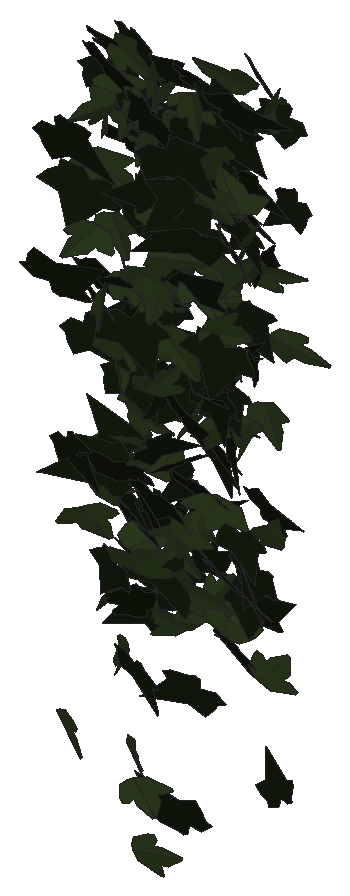
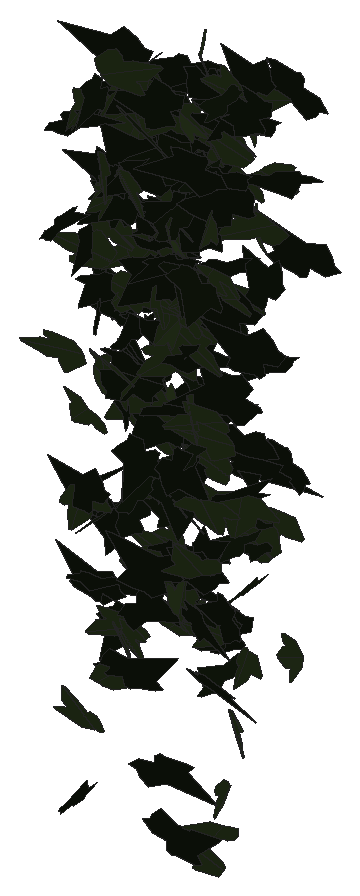
# SketchUp Ruby script. Lengths in millimetres.
U = 1.mm
M = Sketchup.active_model
def pt(a) = Geom::Point3d.new(a.map { |v| v * U })
def face(e, loops, mat)
  f = e.add_face(loops[0].map { |a| pt(a) })
  loops[1..].each { |l| e.add_face(l.map { |a| pt(a) }).erase! }
  f.material = f.back_material = mat if mat
  f
end
# faces: each face lists its corners as indices into pts; further lists are holes
def faces(e, pts, list, mat = nil) = list.each { |f| face(e, (f[0].is_a?(Array) ? f : [f]).map { |l| l.map { |i| pts[i] } }, mat) }
# xy, xz, yz: faces in a plane at the given z, y or x. An outline is a flat list of corners, or four numbers for a rectangle; further outlines are holes
def ring(l) = l.size == 4 ? [[l[0], l[1]], [l[2], l[1]], [l[2], l[3]], [l[0], l[3]]] : l.each_slice(2).to_a
def flat(e, list, mat, &to3) = list.each { |f| face(e, (f[0].is_a?(Array) ? f : [f]).map { |l| ring(l).map { |u, v| to3.(u, v) } }, mat) }
def xy(e, z, list, mat = nil) = flat(e, list, mat) { |x, y| [x, y, z] }
def xz(e, y, list, mat = nil) = flat(e, list, mat) { |x, z| [x, y, z] }
def yz(e, x, list, mat = nil) = flat(e, list, mat) { |y, z| [x, y, z] }
def lines(e, pts, list) = list.each { |a, b| e.add_line(pt(pts[a]), pt(pts[b])) }
# prism: a flat outline (further loops are holes) pulled along v
def prism(e, loops, v, mat = nil)
  f = face(e, loops, mat); d = Geom::Vector3d.new(v.map { |x| x * U })
  f.pushpull(f.normal.samedirection?(d) ? d.length : -d.length)
end
def box(e, o, s, mat = nil) = prism(e, [[o, [o[0] + s[0], o[1], o[2]], [o[0] + s[0], o[1] + s[1], o[2]], [o[0], o[1] + s[1], o[2]]]], [0, 0, s[2]], mat)
def at(x, y, z, deg = 0) = Geom::Transformation.translation(pt([x, y, z])) * Geom::Transformation.rotation(ORIGIN, Z_AXIS, deg.degrees)
def axes(o, x, y, z) = Geom::Transformation.new([*x, 0, *y, 0, *z, 0, *pt(o).to_a, 1])
def part(name) = M.definitions.add(name)
# library, detail: a bought-in or finely detailed component or shape, given as its bounding box
def library(name, o, s) = part(name).tap { |d| box(d.entities, o, s) }
def detail(e, o, s) = box(e.add_group.entities, o, s)
def put(e, d, t, mat = nil) = e.add_instance(d, t).tap { |i| i.material = mat if mat }
def group(e, t, mat = nil) = e.add_group.tap { |g| g.transformation = t; g.material = mat if mat }.entities
root = M.entities
M.materials.add("efeu1").color = [18, 25, 13]
M.materials.add("efeu2").color = [43, 57, 29]
c1 = part("ivyleaf_10")
p = [[0,12.8,-0.8],[-1.5,51.3,-10.9],[-4.9,51,-11.6],[-13.6,26.5,-7.3],[-13.2,15.9,-4.6],[-21.1,19.3,-7.2],
  [-29.5,16.3,-8.3],[-29.2,8.3,-6.2],[-19.7,-9.8,0.5],[-7.6,-13,4],[1,-12.2,5.8],[-0.4,51.1,-11.1],
  [-1.5,51.1,-10.9],[1,-12.4,5.9],[16.9,-12.4,3.5],[35.1,9.1,-5.1],[35,12.9,-6.1],[20.5,16.4,-4.9],
  [15.8,15,-3.8],[15.3,27.6,-7.1],[12.8,31.3,-7.8]]
faces(c1.entities,p,[[0,1,2,3,4,5,6,7,8,9,10],[11,12,0,13,14,15,16,17,18,19,20]],"efeu2")
c2 = part("ivyleaf_9")
p = [[39.1,54.8,31.7],[34.5,51.8,30.2],[-5.3,25.2,17.3],[-17.9,28.3,20.9],[-21.6,21.7,17],[-20.2,4.3,5.3],
  [-22.9,-0.3,2.5],[-17.1,-4,-0.6],[-2,-2.1,-1.2],[-0.7,-15.4,-10.1],[16.6,-22.3,-16.7],[21.1,-15.1,-12.5],
  [32.7,-10.7,-11],[46.1,-1.8,-6.6],[30.8,11.2,3.8]]
faces(c2.entities,p,[[0,1,2,3,4,5,6,7,8,9,10,11,12,13,14]],"efeu1")
put(root,c1,axes([3656.9,861.6,676],[-0.21745,-0.61907,-0.70388],[0.25823,0.6907,-0.6295],[1.76524,-0.1773,0.00538]))
put(root,c2,axes([3619.2,879.4,1196],[0.43031,-0.2889,0.97302],[1.40578,-0.6369,-0.36074],[1.32495,0.76958,0.06673]))
put(root,c2,axes([3622.1,885.5,1606.1],[1.16583,-0.45712,0.56824],[0.91117,-0.30774,-0.76366],[1.04702,0.7768,0.03186]))
put(root,c2,axes([3630,936,783.7],[0.2375,-0.07977,-0.92172],[1.74289,-0.12157,0.1345],[-0.25033,-0.92215,0.062]))
put(root,c1,axes([3628.2,860,1412.2],[1.26885,0.39586,0.80002],[1.29166,0.42377,-0.77526],[-1.10342,0.95128,0.01245]))
put(root,c2,axes([3691.3,953.1,779.3],[-0.34759,0.04433,-0.93711],[-1.77378,0.10065,0.1864],[0.20427,0.94942,0.02399]))
put(root,c1,axes([3663.2,952.2,969.9],[1.67301,0.22774,-0.19223],[-0.3649,-0.02621,-0.9078],[-0.43424,0.89944,0.02222]))
put(root,c1,axes([3666.5,866.2,935.9],[-1.58811,-0.58537,-0.12744],[0.19729,0.07413,-1.01929],[1.12296,-0.84085,-0.00115]))
put(root,c1,axes([3673.5,872.7,571.9],[0.46708,-0.7584,-0.53558],[-0.31943,0.50861,-0.79712],[1.73792,0.29731,-0.00257]))
put(root,c1,axes([3666.9,934.4,1435.8],[0.00493,-0.38442,-0.8398],[0.11088,0.8382,-0.3835],[1.7543,-0.0519,0.0266]))
put(root,c2,axes([3638.2,847.8,875.4],[1.2816,-0.59575,0.122],[0.18383,-0.07494,-0.89907],[1.14267,0.68024,0.00781]))
put(root,c1,axes([3635.4,851.2,863],[-0.96122,-0.02168,0.90204],[1.71102,-0.10013,0.50096],[0.14625,1.02895,0.06776]))
put(root,c2,axes([3671,956.2,1340.8],[0.44979,0.87871,0.40823],[0.22838,0.39042,-0.90984],[-1.82983,0.26472,-0.01321]))
put(root,c2,axes([3687.5,868.9,933.3],[-1.18232,-0.80256,0.2106],[0.27947,0.15259,1.01465],[-1.55421,0.63796,0.02225]))
put(root,c2,axes([3648.9,813.2,1155.2],[0.37024,-0.72384,-0.70986],[-0.01983,0.72135,-0.7384],[1.92942,0.14631,0.12863]))
put(root,c2,axes([3649.4,866.1,1584.9],[-0.1163,-0.61134,-0.73367],[0.43346,0.70463,-0.60611],[1.7651,-0.21332,0.1005]))
put(root,c2,axes([3646.6,773.1,969.1],[-0.38652,-0.0196,-0.94676],[1.8015,0.02388,-0.20354],[0.05227,-0.968,0.01415]))
put(root,c2,axes([3657.1,922.1,1515],[-0.24426,-0.59721,-0.69735],[0.33536,0.67502,-0.61051],[1.71489,-0.21707,0.02006]))
put(root,c2,axes([3645.4,891.3,1130.4],[1.6713,0.14103,0.51566],[0.97157,0.07319,-0.88937],[-0.30206,1.01572,-0.00751]))
put(root,c2,axes([3703.3,907.6,645.4],[-1.69308,0.2827,0.00809],[-0.01696,-0.00134,-0.93343],[-0.53798,-0.88963,0.00397]))
put(root,c2,axes([3687.4,954.7,1351.5],[0.39695,0.8879,0.40846],[0.19909,0.39498,-0.91201],[-1.8494,0.2331,-0.01051]))
put(root,c1,axes([3649.4,936.1,1074.4],[-0.21937,-0.08976,-0.936],[1.77507,-0.13076,-0.10232],[-0.22743,-0.93397,0.10429]))
put(root,c1,axes([3662.9,916.4,735.4],[0.85517,0.18966,-0.7966],[1.12189,0.55578,0.46483],[1.08175,-0.72634,0.14767]))
put(root,c2,axes([3661.9,905.7,1623],[0.65898,-0.84368,0.2148],[0.1378,-0.20245,-0.91192],[1.65117,0.35361,-0.00962]))
put(root,c2,axes([3655.9,722.2,1275.2],[-0.47995,0.04865,1.02424],[1.56186,-0.62281,0.23164],[1.17005,0.85133,0.11093]))
put(root,c2,axes([3686.8,771,1434.7],[-1.28367,-0.88403,-0.01548],[0.0178,0.01233,-1.11195],[1.68265,-0.67454,-0.00004]))
put(root,c2,axes([3659,964.6,1541.7],[0.20429,0.13717,-0.89428],[1.09147,0.6862,0.17409],[1.33178,-0.58343,-0.0055]))
put(root,c2,axes([3664.1,863.8,865.9],[0.7315,-0.89886,0.23349],[0.23371,-0.20129,-0.97703],[1.75196,0.40216,0.03285]))
put(root,c1,axes([3682.6,770.3,862.1],[-1.35554,-0.58375,-0.47634],[0.76287,0.26145,-0.91974],[1.21417,-0.81599,0.04607]))
put(root,c2,axes([3729.3,792,946.7],[-1.83934,-0.13213,0.57145],[-1.07745,-0.0778,-0.97544],[0.29182,-1.12005,0.00034]))
put(root,c1,axes([3665.9,934.9,1102.2],[0.61249,0.27061,0.85149],[1.14987,0.60083,-0.4193],[-1.25271,0.68382,0.03144]))
put(root,c1,axes([3677.7,951.3,856.5],[1.28464,0.44572,-0.49084],[0.78541,0.26579,0.80886],[0.98762,-0.79113,-0.00479]))
put(root,c2,axes([3704.5,973,1036.4],[-0.4994,0.64473,-0.79081],[0.56615,-0.73273,-0.69608],[-1.85752,-0.39666,0.00046]))
put(root,c1,axes([3702.2,792.3,1564.2],[0.02712,-0.18041,1.09376],[-0.03713,-1.09372,-0.18015],[2.10945,-0.01693,-0.01723]))
put(root,c2,axes([3664.1,895.3,1439.8],[1.99242,0.11403,-0.23279],[0.43455,0.05293,1.05272],[0.23357,-1.07114,0.02724]))
put(root,c1,axes([3692.4,844.7,1098],[-0.04657,0.87777,-0.46591],[0.00724,-0.46597,-0.87807],[-1.8913,-0.0234,0.00811]))
put(root,c2,axes([3671.8,824,1610.1],[0.1947,-0.36131,0.95831],[0.7325,-0.87892,-0.37247],[1.80631,0.39537,0.04775]))
put(root,c1,axes([3676,848.3,1570.1],[1.23771,0.43203,0.5737],[0.9251,0.30496,-0.78066],[-1.00619,0.81182,-0.01205]))
put(root,c1,axes([3683.2,814.1,1532.5],[-0.20584,0.08717,0.99849],[1.16609,-0.78903,0.13525],[1.50962,0.62137,0.03167]))
put(root,c2,axes([3685.5,938.1,1499.9],[-0.06883,-0.70313,0.65646],[0.13713,-0.65706,-0.6998],[1.82563,0.02284,0.07732]))
put(root,c1,axes([3695.4,921.7,1306],[0.0097,0.27879,0.91595],[0.05528,0.9155,-0.27881],[-1.82136,0.02927,-0.00358]))
put(root,c1,axes([3706.7,931.7,1114],[0.35004,-0.95221,-0.29135],[-0.01287,0.29508,-0.96866],[1.89514,0.17788,0.04724]))
put(root,c2,axes([3699.2,821.4,751.9],[-0.36075,-0.63647,0.63104],[-0.27021,-0.61553,-0.66348],[1.68425,-0.23508,0.02872]))
put(root,c1,axes([3672.8,865.5,1620.4],[0.52665,-0.04353,0.97521],[1.8006,-0.23776,-0.27907],[0.4577,0.98543,-0.02426]))
put(root,c1,axes([3740.6,906.9,1202.3],[-1.08951,0.04027,0.78396],[-1.49041,-0.0966,-0.56687],[0.10363,-0.96591,0.08937]))
put(root,c2,axes([3676.7,896.9,723.2],[0.67271,-0.64871,0.71095],[0.73097,-0.59938,-0.73786],[1.67952,0.5207,0.03638]))
put(root,c2,axes([3693.9,855.8,1072.6],[0.16033,-0.92547,-0.48982],[-0.09594,0.48724,-0.92928],[1.99053,0.09803,-0.00534]))
put(root,c1,axes([3711.4,847.1,428],[-0.78238,0.78469,0.13375],[-0.12398,0.11687,-0.88585],[-1.50989,-0.4162,0.00343]))
put(root,c2,axes([3732.9,912.1,1182.4],[-0.12547,-0.31972,-0.89004],[-0.34126,-0.8718,0.32644],[-1.76726,0.19104,0.00015]))
put(root,c2,axes([3690.2,945.3,1040.6],[0.81623,-0.84097,0.0972],[0.08586,-0.0861,-0.94402],[1.60891,0.43124,0.00106]))
put(root,c2,axes([3688.9,776.2,1239.5],[0.16706,-0.43073,1.07078],[0.44133,-1.0454,-0.43952],[2.15182,0.24785,0.00701]))
put(root,c1,axes([3677.6,863.5,1518.4],[0.8567,-0.25701,-1.03394],[1.92297,-0.25306,0.50279],[-0.64319,-1.09892,0.12603]))
put(root,c2,axes([3742.3,870.1,1549.8],[-0.28626,-0.38716,-0.88076],[-0.404,-0.85613,0.41259],[-1.78594,0.25572,0.04784]))
put(root,c1,axes([3718,831.1,1541.5],[1.22018,-0.65683,0.09752],[0.12784,-0.07071,-0.91786],[1.2573,0.64463,-0.00131]))
put(root,c2,axes([3730.5,793.1,1187.6],[0.14784,0.5784,0.83399],[0.2192,0.826,-0.58359],[-1.91914,0.1389,-0.00241]))
put(root,c2,axes([3737.7,866.9,819.1],[0.10398,-0.51843,0.78811],[-0.23867,0.77843,0.52076],[-1.77943,-0.13471,-0.02379]))
put(root,c2,axes([3684.4,702.3,1555],[-0.00715,-0.1984,-1.09862],[2.03355,0.31772,-0.06103],[0.6157,-1.05168,0.18881]))
put(root,c2,axes([3706.5,970.2,1374.1],[0.2403,-0.54117,-0.7389],[0.10151,0.74896,-0.53943],[1.74014,0.03104,0.1335]))
put(root,c1,axes([3719.6,867,1484],[1.28921,-0.66424,0.18482],[0.25333,-0.12824,-0.94872],[1.28753,0.69034,0.0016]))
put(root,c1,axes([3694.3,877.1,986.3],[-0.29166,-0.01332,0.92108],[1.73339,-0.1421,0.14948],[0.26269,0.92287,0.03631]))
put(root,c2,axes([3755,950.4,501.9],[0.1189,0.05227,-0.90793],[-1.14396,-0.68058,-0.08054],[-1.29889,0.60419,-0.01218]))
put(root,c1,axes([3718.9,852.3,362.4],[0.99501,0.70498,0.2678],[0.30626,0.21407,-0.87768],[-1.4022,0.54701,-0.00166]))
put(root,c1,axes([3742.6,710.9,1393.5],[0.95573,0.5619,-0.68683],[-0.86734,-0.51386,-0.7536],[-1.44916,0.67813,-0.00193]))
put(root,c2,axes([3743.1,762.5,972.7],[1.20316,0.47432,-0.58118],[-0.94156,-0.30772,-0.78927],[-1.07323,0.80171,0.0409]))
put(root,c2,axes([3707.1,829,685.7],[0.5167,0.13056,0.96082],[1.67519,0.38541,-0.30108],[-0.77421,0.92106,-0.01021]))
put(root,c2,axes([3698.1,837.8,1218.7],[0.45884,-0.31901,0.88483],[1.58674,-0.35039,-0.35349],[0.82872,0.84751,0.18692]))
put(root,c1,axes([3708.8,932.5,1260.6],[0.81864,-0.26362,0.82798],[1.42902,-0.35223,-0.50222],[0.83236,0.86401,0.04788]))
put(root,c2,axes([3721.4,818.4,1539.9],[-0.30029,-0.37145,1.00974],[0.45217,-1.00738,-0.33346],[1.9971,0.17223,0.22733]))
put(root,c1,axes([3711,831.2,1246.6],[1.2725,-0.0808,0.79441],[1.48718,-0.14706,-0.67263],[0.31281,1.02786,-0.03379]))
put(root,c1,axes([3747.6,889.2,1563.8],[0.23451,-0.74909,0.5757],[0.11873,-0.57286,-0.75874],[1.79414,0.13582,-0.02504]))
put(root,c1,axes([3729.5,659.8,566.7],[-0.64757,0.59912,-0.75382],[0.69556,-0.65932,-0.68898],[-1.69547,-0.49931,0.00526]))
put(root,c2,axes([3721.7,888.7,820.6],[0.08344,0.08836,-0.92981],[0.71746,0.84997,0.09855],[1.62636,-0.37949,0.00423]))
put(root,c1,axes([3750.5,920.5,1383.6],[0.41925,-0.89383,0.28163],[0.11971,-0.27456,-0.92056],[1.77955,0.22905,-0.00443]))
put(root,c1,axes([3747,928.5,1236.7],[-1.09791,0.82919,-0.27494],[0.29823,-0.22591,-1.01012],[-1.63563,-0.59778,0.00037]))
put(root,c1,axes([3736,849.1,1490.3],[1.49151,-0.6692,-0.46399],[0.66722,-0.30397,1.03052],[-1.39883,-0.85852,-0.00319]))
put(root,c1,axes([3753.1,834.9,1272.3],[-1.61102,-0.36436,-0.32955],[0.57942,0.12624,-0.92156],[0.73385,-0.89955,0.00415]))
put(root,c2,axes([3735.8,821.3,594.1],[0.41582,-0.9221,0.46101],[0.19404,-0.44961,-0.94763],[1.95243,0.24107,-0.004]))
put(root,c1,axes([3749.3,762,1374.7],[-0.50796,0.69229,-0.65388],[0.36154,-0.62672,-0.74107],[-1.77593,-0.3256,0.03616]))
put(root,c1,axes([3755.7,902.6,744.8],[-0.10166,-0.47538,-0.88061],[-0.03343,-0.88128,0.47681],[-1.9043,0.04085,0.03864]))
put(root,c2,axes([3768.7,883.7,926.8],[0.41479,0.94679,0.11276],[0.03892,0.111,-0.97154],[-1.81424,0.21884,0.00494]))
put(root,c1,axes([3741.7,905,1325.1],[1.89026,-0.30287,0.44265],[0.81669,-0.11015,-1.0382],[0.61239,1.08178,0.01822]))
put(root,c2,axes([3717.5,894.2,1399.2],[0.75362,0.27725,-1.01789],[1.59682,0.57633,0.48338],[1.21717,-0.92776,-0.00391]))
put(root,c2,axes([3786.3,796.4,1575.6],[0.76973,0.00846,-1.01913],[-1.93967,0.00164,-0.40444],[-0.00304,1.09644,0.00847]))
put(root,c2,axes([3739.4,923.6,1398.6],[0.58563,-0.69708,0.52633],[0.41371,-0.47936,-0.76196],[1.61007,0.37672,0.00434]))
put(root,c1,axes([3769.7,917.7,1274.3],[-0.36004,-0.92063,-0.22612],[0.11983,0.21787,-0.9397],[1.80023,-0.19863,0.01733]))
put(root,c2,axes([3800.8,866.2,323],[0.12066,-0.10933,0.99298],[-1.29977,0.72142,0.12303],[-1.38759,-0.68527,-0.0289]))
put(root,c2,axes([3754.6,858.1,1499.3],[-1.13837,-0.1485,0.98807],[1.90109,-0.06188,0.59539],[-0.04458,1.15335,0.15916]))
put(root,c1,axes([3751.1,749,1397.8],[1.39782,-0.27727,0.58688],[1.06264,-0.18206,-0.78476],[0.62997,0.92234,0.02152]))
put(root,c1,axes([3743,751.9,1194.8],[-0.17296,-0.06928,-1.08662],[1.849,0.48718,-0.11231],[0.93566,-0.97553,0.02108]))
put(root,c1,axes([3777.6,861.5,722.4],[0.10615,-0.79808,0.65077],[0.15275,-0.64637,-0.79956],[1.9539,0.09389,0.02715]))
put(root,c1,axes([3761.3,709.3,1291.1],[0.66115,-0.49754,0.88006],[0.95289,-0.72376,-0.60681],[1.67153,0.60939,-0.00217]))
put(root,c2,axes([3756.8,852.7,1334.8],[-0.35548,-0.10082,1.13534],[1.96893,0.46791,0.21175],[-0.91054,1.05116,0.01463]))
put(root,c2,axes([3816.1,833.1,743.7],[-0.865,-0.08174,-0.8077],[-1.46686,-0.24731,0.45873],[-0.48531,0.89318,0.0531]))
put(root,c2,axes([3751.2,946.1,813.8],[1.42099,0.59788,-0.11369],[0.15154,0.08243,0.9564],[1.14831,-0.75072,0.01447]))
put(root,c2,axes([3746.3,908.9,1498.9],[1.49367,-0.52143,0.29815],[0.48619,-0.15422,-0.94217],[1.03461,0.82526,0.01231]))
put(root,c2,axes([3802.8,900.7,1340.1],[-1.79765,-0.17449,0.08848],[-0.16311,-0.02313,-0.96049],[0.33472,-0.94839,0.00715]))
put(root,c2,axes([3794.2,807,1064.1],[0.03769,0.67615,0.64512],[0.04457,0.64471,-0.67643],[-1.77806,0.03049,-0.00328]))
put(root,c1,axes([3757.2,896,1376.4],[1.06795,-0.29933,0.71909],[1.2996,-0.2373,-0.63163],[0.71312,0.88071,0.07421]))
put(root,c2,axes([3807.9,961.2,638],[0.40135,0.02513,0.89081],[-1.6827,0.12062,0.2059],[-0.21256,-0.90745,0.05204]))
put(root,c2,axes([3801,868.5,1430.7],[0.98805,-0.09717,0.82242],[-1.50863,0.22268,0.52669],[-0.45625,-0.94673,0.03947]))
put(root,c1,axes([3785.1,789.7,1003.3],[-0.00983,0.11546,-1.04342],[-0.30858,-1.031,-0.11329],[-1.97398,0.1606,0.02291]))
put(root,c2,axes([3793,887.5,1062.7],[-1.17091,-0.78409,0.31422],[-0.37355,-0.24539,-0.99665],[1.56365,-0.64578,-0.0028]))
put(root,c2,axes([3799.9,871.9,914.6],[-1.41816,0.47072,-0.34018],[0.55528,-0.17508,-0.88135],[-0.95574,-0.8002,-0.00727]))
put(root,c2,axes([3768.2,915.7,1301.4],[1.74666,0.25049,0.0307],[0.05382,0.01301,-0.95131],[-0.47727,0.91817,0.0051]))
put(root,c2,axes([3796.6,941.6,754.8],[-0.16558,0.09537,-0.95392],[0.39641,-0.93308,-0.11228],[-1.78098,-0.21655,0.0637]))
put(root,c1,axes([3756.8,819.3,279],[0.54152,-0.18791,-0.84865],[1.42622,-0.39941,0.33969],[-0.83817,-0.80103,0.02971]))
put(root,c1,axes([3774,808.7,1511.5],[-0.00544,-0.46987,0.95246],[1.08637,-0.80388,-0.39486],[1.70454,0.51084,0.2547]))
put(root,c1,axes([3808.8,841.6,675.1],[-0.95554,-0.41287,-0.63439],[-0.88688,-0.43128,0.64949],[-1.13518,0.68449,0.02657]))
put(root,c1,axes([3772.8,819,1626.2],[0.43991,-0.45617,0.968],[1.22269,-0.73284,-0.49876],[1.62875,0.67334,0.11297]))
put(root,c1,axes([3782.2,876.6,1146.4],[-1.15303,-0.36888,-0.63161],[1.02886,0.32663,-0.7093],[0.93772,-0.81196,0.00161]))
put(root,c1,axes([3835,921.1,1263.2],[0.26044,-0.05826,-1.04865],[-1.85896,0.38164,-0.14866],[0.73471,0.98628,-0.00442]))
put(root,c1,axes([3799.1,858.8,1368.4],[0.30007,-0.33656,-1.00353],[0.39543,1.0047,-0.30431],[1.97527,-0.15,0.21337]))
put(root,c1,axes([3784.6,894.7,1554.2],[1.46577,0.36223,0.37402],[0.62196,0.1836,-0.85073],[-0.77145,0.83626,0.02477]))
put(root,c1,axes([3816.2,948.8,1463.5],[0.85738,-0.58358,-0.58199],[-0.59283,0.4935,-0.73596],[1.45223,0.54599,0.04316]))
put(root,c2,axes([3767.3,912.2,1579.7],[1.16145,-0.48236,0.58631],[0.91192,-0.33882,-0.77747],[1.12086,0.77549,0.025]))
put(root,c2,axes([3834.2,910.7,1539.3],[-1.05066,0.73691,0.32359],[-0.3916,0.25013,-0.92065],[-1.48084,-0.58898,0.01387]))
put(root,c2,axes([3791,744.6,1241.1],[-0.42331,-0.97151,-0.4687],[0.22022,0.45431,-0.99659],[2.04106,-0.25051,0.01032]))
put(root,c1,axes([3797.3,750.7,817.7],[-1.52419,-0.49624,0.46193],[0.76967,0.22415,0.94192],[-1.0356,0.89694,0.02018]))
put(root,c2,axes([3841,733.9,1487.6],[-1.29827,0.69304,0.19759],[-0.26356,0.14094,-0.97244],[-1.34599,-0.69606,-0.00017]))
put(root,c2,axes([3790.9,814.3,1515],[-0.12783,0.05527,-1.07583],[1.81147,-0.50179,-0.0852],[-0.96021,-0.95401,-0.01751]))
put(root,c2,axes([3800.7,818.6,792.2],[-0.78912,-0.79078,-0.5533],[0.48543,0.49101,-0.89289],[1.77154,-0.48679,-0.0018]))
put(root,c2,axes([3819.6,831.8,1362.7],[-1.77273,-0.41684,-0.35993],[0.61705,0.15662,-1.02042],[0.84728,-0.98621,-0.00992]))
put(root,c2,axes([3822.8,759.4,945.5],[1.36477,0.05236,-0.68362],[-1.30218,-0.00897,-0.71839],[-0.08392,0.9907,0.02963]))
put(root,c2,axes([3804.1,898.2,1459.5],[0.18378,-0.20229,-1.02126],[-0.02038,1.0254,-0.20412],[1.98133,0.02931,0.09263]))
put(root,c1,axes([3812,770.2,1123.3],[-0.84202,-0.72861,0.42578],[0.42556,0.36235,0.85241],[-1.5487,0.49571,0.00274]))
put(root,c1,axes([3836.3,963.8,624.1],[0.53731,0.65238,0.63256],[-0.47276,-0.58175,0.71084],[1.66356,-0.37604,-0.0023]))
put(root,c2,axes([3814.6,760.8,1024],[0.06073,0.40173,-0.86173],[-0.26176,0.85509,0.39354],[1.79046,0.11138,0.08676]))
put(root,c2,axes([3822.4,897.5,978.3],[1.56388,-0.16314,-0.62354],[-1.14806,0.16117,-0.83712],[0.43204,1.01884,0.03258]))
put(root,c2,axes([3806,936.1,924.3],[0.19276,-0.72727,0.75792],[0.14411,-0.7544,-0.73401],[1.99394,0.12483,-0.02022]))
put(root,c2,axes([3804.5,774.2,1447.6],[-0.13657,-0.43035,-1.09772],[0.42281,1.07512,-0.43602],[2.20381,-0.23294,0.01562]))
put(root,c1,axes([3816.3,815.6,1360.8],[-1.79225,0.08484,0.47864],[0.86112,-0.22848,0.93069],[0.3382,1.03136,0.1668]))
put(root,c1,axes([3799,840.1,808.6],[0.52476,-0.08015,0.86159],[1.52747,-0.31435,-0.28608],[0.61563,0.84826,-0.02461]))
put(root,c1,axes([3842.6,931.7,698],[1.39326,-0.45223,-0.41717],[-0.66648,0.22685,-0.86044],[0.96278,0.81147,0.00805]))
put(root,c1,axes([3824.8,835,1026.7],[0.32151,-1.03066,0.09364],[0.03669,0.09799,1.04384],[-1.96929,-0.16644,0.03473]))
put(root,c1,axes([3813.1,860.8,1574.9],[1.12259,-0.44215,0.64999],[1.01012,-0.37546,-0.73704],[1.10368,0.79337,0.01344]))
put(root,c1,axes([3837.1,936.7,692],[0.82537,-0.85625,0.09704],[0.08077,-0.08728,-0.95981],[1.63805,0.43574,-0.00157]))
put(root,c2,axes([3808.1,833.4,859.3],[0.79669,-0.72926,0.48341],[0.43673,-0.42562,-0.84079],[1.60688,0.47724,-0.01115]))
put(root,c1,axes([3869.7,909.7,1607.4],[-0.97394,0.01002,-0.83275],[-1.56906,-0.14439,0.50489],[-0.22427,0.9667,0.08404]))
put(root,c1,axes([3818.4,755,1441],[0.44861,0.2544,0.92554],[0.7208,0.85106,-0.33038],[-1.6786,0.43344,0.10549]))
put(root,c1,axes([3817.1,781.3,1346.5],[-0.3429,-0.09049,-1.02991],[1.57798,0.61188,-0.19881],[1.17546,-0.84781,-0.03356]))
put(root,c1,axes([3855.8,802.4,875.2],[-1.31871,-0.8151,0.09386],[-0.11055,-0.07381,-1.0698],[1.55763,-0.69531,0.00354]))
put(root,c1,axes([3816,816.8,1450.6],[-0.04267,-0.07069,0.94311],[1.77181,0.16452,0.03446],[-0.31705,0.92892,0.06566]))
put(root,c2,axes([3850.4,851.8,1168.6],[-1.47093,-0.4206,-0.38923],[0.67434,0.1629,-0.87958],[0.85721,-0.84988,0.02403]))
put(root,c1,axes([3821.8,931.3,702.7],[0.9225,0.28103,0.77164],[1.26922,0.38819,-0.56029],[-0.91209,0.82443,0.00078]))
put(root,c1,axes([3859.7,948.7,1475.2],[0.6213,-0.72806,-0.74673],[-0.21845,0.75262,-0.78398],[1.97282,0.31263,0.14836]))
put(root,c1,axes([3865.1,830.1,737],[1.53439,-0.12206,-0.46029],[-0.86928,0.05783,-0.81535],[0.25639,0.92656,-0.00975]))
put(root,c2,axes([3840.8,895.4,1465.8],[-0.72467,-0.29723,0.91157],[1.65615,0.30469,0.46283],[-0.76617,0.93974,0.13826]))
put(root,c1,axes([3858.5,903,1228.4],[-0.21404,0.46146,0.98257],[0.3002,-0.9704,0.4738],[2.04407,0.19084,0.0333]))
put(root,c2,axes([3855.2,961.9,1605.5],[1.22796,-0.34861,-0.57771],[-0.96554,0.27636,-0.73337],[0.84666,0.82078,0.00155]))
put(root,c2,axes([3845.5,870.9,1607.7],[0.61772,-0.86849,-0.30593],[-0.24554,0.27829,-0.92689],[1.73518,0.34856,-0.02225]))
put(root,c1,axes([3829.6,780,1211.2],[1.61744,0.03534,0.75846],[1.43923,0.06284,-0.85027],[-0.12978,1.13735,0.02341]))
put(root,c2,axes([3841.1,818.5,1281.7],[-0.65191,-0.15034,1.01336],[1.35303,-0.80423,0.12099],[1.40385,0.7053,0.35397]))
put(root,c2,axes([3851.1,905.7,1399.4],[1.75246,-0.25463,-0.12738],[-0.23524,0.03093,-0.95535],[0.48815,0.92905,-0.00311]))
put(root,c1,axes([3837.2,815.8,760.5],[-0.52238,-0.00104,1.01632],[1.92316,-0.11287,0.27278],[0.20687,1.04666,0.03043]))
put(root,c2,axes([3854.6,752.1,1555.7],[-0.06832,-0.626,-0.94105],[0.19735,0.93573,-0.62642],[2.14201,-0.10618,0.0277]))
put(root,c1,axes([3875.6,858.5,1035.7],[-0.05774,0.29409,1.10951],[0.24239,-1.10218,0.29563],[2.17105,0.13088,-0.0035]))
put(root,c2,axes([3849.7,797.3,1070],[-0.03871,-0.27964,1.0367],[0.63543,-0.98714,-0.25972],[1.94227,0.31738,0.10563]))
put(root,c1,axes([3859.6,828.4,1288],[1.31582,0.68912,0.2772],[0.37714,0.19386,-0.97616],[-1.36244,0.71921,-0.00249]))
put(root,c1,axes([3880.9,816,1532.5],[-1.28131,-0.77958,-0.18345],[0.22317,0.14112,-1.03004],[1.50779,-0.68337,-0.00343]))
put(root,c1,axes([3882,902.8,1389.2],[0.16541,-0.12552,1.04397],[-0.46608,1.01631,0.14259],[-1.94617,-0.25406,0.05458]))
put(root,c1,axes([3875,837.4,754.8],[0.19471,0.30324,-0.85805],[0.47382,0.8212,0.31989],[1.66596,-0.269,0.00931]))
put(root,c2,axes([3863.9,864,1098.4],[-0.88392,-0.29987,-0.73908],[1.31996,0.27053,-0.54559],[0.74965,-0.82991,0.0892]))
put(root,c2,axes([3867.2,867.5,1054.4],[1.76505,-0.50843,-0.01362],[0.03373,0.00399,1.05757],[-0.9674,-0.9275,0.01202]))
put(root,c2,axes([3885.7,847.4,1128],[-0.67351,-0.51689,0.85583],[0.9552,0.69335,0.62628],[-1.64573,0.61396,0.01325]))
put(root,c1,axes([3878.1,867.5,1415.6],[-0.18516,-0.3833,-0.94649],[0.52663,0.90531,-0.39506],[1.87075,-0.29279,0.01753]))
put(root,c1,axes([3881,903.1,1559.4],[-0.49676,0.92977,0.09922],[-0.06144,0.09399,-0.9657],[-1.77853,-0.26294,0.00564]))
put(root,c1,axes([3879.8,876.4,1386.5],[0.2063,-0.56668,0.81481],[-0.09077,0.81573,0.57367],[-1.88673,-0.10121,0.06149]))
put(root,c1,axes([3864,979.5,549.9],[1.56976,-0.33355,-0.39557],[0.71526,-0.12546,0.88941],[-0.67689,-0.90611,0.02247]))
put(root,c2,axes([3878,867.9,665.3],[1.54929,-0.21703,-0.46569],[-0.85581,0.12109,-0.84248],[0.47299,0.92998,0.00102]))
put(root,c2,axes([3872,786.4,970.9],[1.8701,-0.09894,-0.30044],[-0.56665,0.04177,-0.98751],[0.20328,1.02666,0.01122]))
put(root,c1,axes([3887.9,849.3,1477.8],[-1.18401,0.76455,-0.06126],[0.067,-0.05034,-0.98567],[-1.45821,-0.62309,0.00445]))
put(root,c1,axes([3874.6,793.8,1468.4],[-1.53357,-0.27829,-0.64718],[1.15259,0.2287,-0.85236],[0.68496,-1.00789,-0.01471]))
put(root,c2,axes([3871.5,862.7,1548.3],[-0.50476,-0.36564,-0.8787],[0.91601,0.73541,-0.45128],[1.56265,-0.5492,-0.01929]))
put(root,c2,axes([3879.9,843.6,1095.2],[-0.83894,0.00348,-0.78847],[1.48223,-0.13913,-0.43602],[-0.23432,-0.89255,0.06489]))
put(root,c1,axes([3903.9,941.7,1552.4],[-0.03898,0.12056,1.09236],[-0.74979,1.01913,-0.11986],[-1.95258,-0.39375,0.02422]))
put(root,c2,axes([3893,899.9,1367.4],[-0.23905,-0.46272,0.84173],[-0.50268,-0.79953,-0.47894],[1.75762,-0.2916,-0.02249]))
put(root,c1,axes([3890.9,681.9,1357],[1.61684,-0.58492,0.13821],[0.2192,-0.07643,-1.03142],[1.12267,0.85731,0.00235]))
put(root,c2,axes([3924.1,738.9,1439.7],[0.1511,0.12689,-1.04983],[-0.96196,-0.92019,-0.14944],[-1.7678,0.51157,-0.00841]))
put(root,c2,axes([3912.6,967.7,1537.6],[-0.00451,-0.43186,-0.83523],[-0.08607,-0.83421,0.43147],[-1.78746,0.04126,-0.01867]))
put(root,c2,axes([3910.4,740.7,1490.3],[-1.24041,-0.72254,0.59603],[-0.64831,-0.49356,-0.9708],[1.66057,-0.73241,0.06621]))
put(root,c1,axes([3884.1,758.2,900.8],[1.56574,-0.43799,-0.23201],[0.3996,-0.09929,0.93195],[-0.85449,-0.84899,0.0107]))
put(root,c2,axes([3915,731.8,1495.6],[-0.97398,0.84528,-0.61778],[0.61837,-0.52547,-0.98812],[-1.89423,-0.60617,-0.00492]))
put(root,c2,axes([3895.9,902.9,742.8],[-1.22886,-0.59114,-0.3949],[0.55577,0.26585,-0.87541],[1.23359,-0.70865,0.00101]))
put(root,c2,axes([3869,914.5,1436.9],[0.55673,-0.18727,-0.87388],[1.69985,0.09395,0.27884],[0.06047,-0.91674,0.20709]))
put(root,c2,axes([3889.5,875.9,1234.4],[-0.37421,-0.63344,-0.76609],[0.45982,0.72707,-0.66318],[1.83516,-0.31134,0.00995]))
put(root,c2,axes([3913.3,905.4,1313.9],[-0.02639,0.03621,-0.93856],[-1.03108,0.76647,0.03757],[1.46026,0.54186,0.00957]))
put(root,c2,axes([3894.6,864.3,1336.2],[-0.40202,-0.0947,1.08472],[0.1615,-1.10301,-0.07977],[2.06599,0.06779,0.21731]))
put(root,c2,axes([3908.1,996.4,1376.6],[0.22048,-0.36386,-0.85317],[0.64852,-0.78298,0.38019],[-1.64182,-0.35814,0.0356]))
put(root,c2,axes([3919.5,943.8,376.9],[-0.64317,-0.61115,0.6123],[0.56729,0.53485,0.69836],[-1.54566,0.45061,0.00153]))
put(root,c1,axes([3920.7,863.8,1323.2],[-0.34342,-0.94428,0.55322],[-0.17786,-0.54535,-0.96132],[2.07525,-0.203,0.00916]))
put(root,c1,axes([3915.9,825.5,1194],[-0.66109,0.89838,0.34334],[-0.26133,0.31498,-0.9631],[-1.81166,-0.37326,0.01364]))
put(root,c2,axes([3896.2,850.8,1029.5],[-0.3281,0.11665,-1.07675],[1.86174,-0.4512,-0.2055],[-0.88471,-0.99274,-0.03312]))
put(root,c2,axes([3894.6,834,1169.7],[1.26403,0.72675,0.15353],[-0.20587,-0.10913,0.9845],[1.39862,-0.67289,0.00616]))
put(root,c1,axes([3889,857.3,1054.9],[0.39654,-0.37853,-0.86078],[1.34809,-0.5167,0.39867],[-1.17707,-0.71929,0.16661]))
put(root,c2,axes([3899.1,870.7,1392.4],[0.34208,-0.9474,0.35065],[0.16857,-0.34001,-0.96405],[1.91523,0.19914,0.02222]))
put(root,c1,axes([3898.9,934.5,1039.2],[1.3947,-0.25754,0.60784],[1.07615,-0.22381,-0.77653],[0.64841,0.92542,-0.01865]))
put(root,c1,axes([3930.9,824.2,1459.5],[1.75491,0.17737,0.33075],[-0.62626,-0.03982,0.93874],[0.3435,-0.9788,0.02174]))
put(root,c1,axes([3914.6,788,1245.3],[0.33705,0.37383,1.08122],[0.16841,1.08635,-0.3901],[-2.17079,0.14232,0.13761]))
put(root,c1,axes([3935.1,773.5,959.2],[1.52751,0.49068,-0.51447],[-0.83836,-0.2658,-0.94071],[-1.06206,0.91553,0.00262]))
put(root,c1,axes([3926.3,863.7,1385.6],[0.60032,-0.95193,0.48554],[0.30614,-0.45819,-1.0028],[2.01061,0.35399,0.00771]))
put(root,c2,axes([3924.1,881.6,1154.3],[-0.07359,0.24922,1.07237],[-0.61722,-1.028,0.22721],[2.00235,-0.30772,0.10945]))
put(root,c2,axes([3890.2,848.8,1594.7],[0.60202,-0.17335,0.9208],[1.52395,-0.45466,-0.36067],[0.92603,0.86093,-0.00507]))
put(root,c1,axes([3899.2,910.3,1290.6],[-0.43042,-0.30676,0.88598],[1.51048,0.42261,0.34891],[-0.95005,0.81088,0.15333]))
put(root,c2,axes([3898.1,821,808.8],[1.15078,-0.65906,0.42677],[0.57694,-0.30094,-0.89423],[1.37848,0.67615,0.01798]))
put(root,c2,axes([3907.2,893.2,716.4],[-0.29061,0.13015,0.90461],[1.15825,-0.66976,0.19909],[1.29766,0.62695,0.02489]))
put(root,c1,axes([3936.4,896.7,868.1],[-0.8464,-0.82261,-0.42579],[0.40838,0.36799,-0.93504],[1.71493,-0.49363,0.01251]))
put(root,c2,axes([3907.8,917,881.4],[0.3177,-0.27808,0.91196],[0.87445,-0.78777,-0.32431],[1.58993,0.48883,-0.00386]))
put(root,c2,axes([3936.2,787.5,1225.5],[-0.91611,-0.97775,0.09544],[-0.07895,-0.08596,-1.08982],[1.86804,-0.48313,0.00075]))
put(root,c1,axes([3908.5,964.5,1149.8],[-0.50105,0.0019,-0.89513],[1.67165,-0.17937,-0.25871],[-0.32852,-0.91564,0.04882]))
put(root,c1,axes([3939.7,852.8,1057],[0.24817,-0.68343,0.67365],[0.36993,-0.64694,-0.69396],[1.78851,0.22864,0.05006]))
put(root,c2,axes([3915.5,852.3,804.2],[0.16566,-0.00215,-1.04786],[1.86205,-0.37635,0.08204],[-0.71414,-0.98181,-0.02915]))
put(root,c2,axes([3931,832.4,881.3],[-0.02126,-0.90154,-0.05999],[0.00934,0.05993,-0.9016],[1.71958,-0.01147,0.00415]))
put(root,c2,axes([3940.8,864.7,809.7],[-0.3595,-0.82239,0.63797],[-0.29753,-0.61862,-0.84374],[1.95844,-0.24494,-0.01108]))
